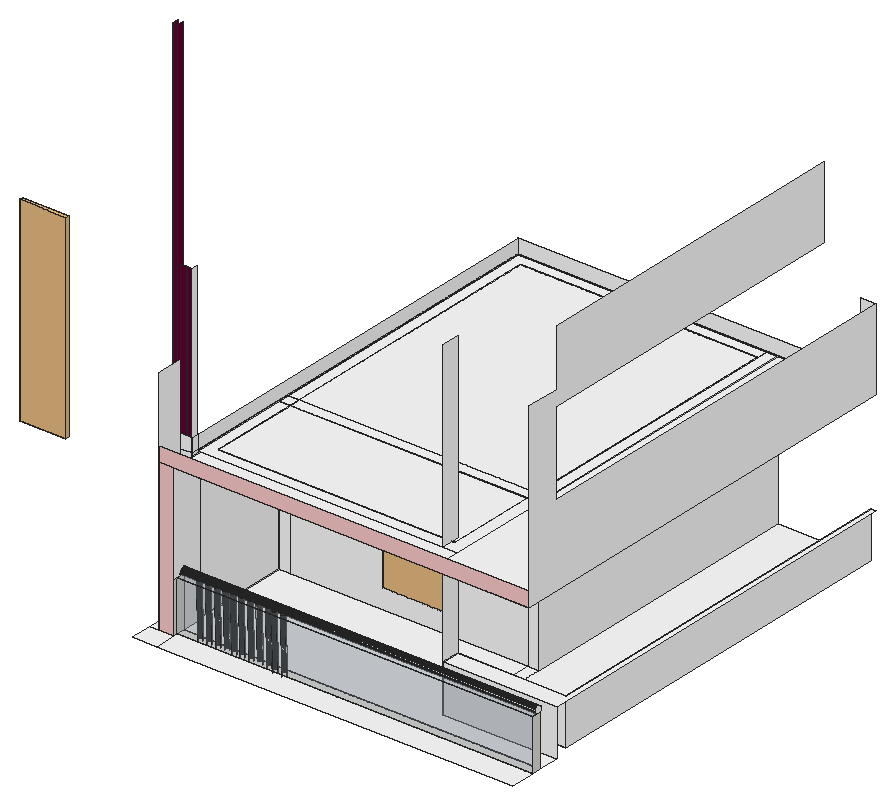
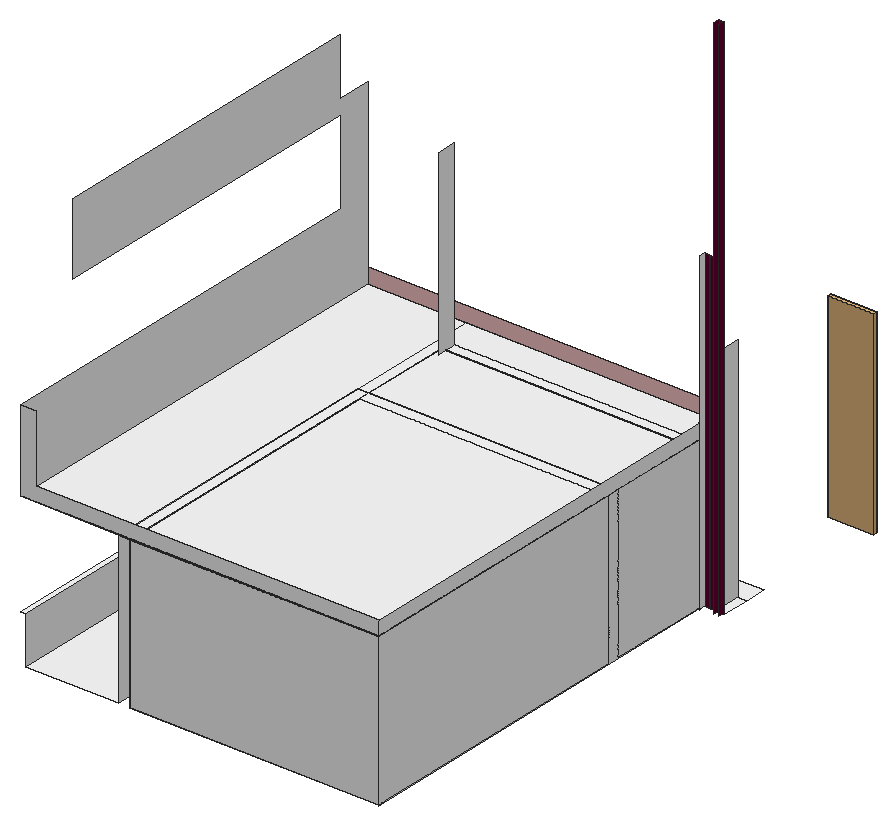
# SketchUp Ruby script. Lengths in inches.
U = 1.inch
M = Sketchup.active_model
def pt(a) = Geom::Point3d.new(a.map { |v| v * U })
def face(e, loops, mat)
  f = e.add_face(loops[0].map { |a| pt(a) })
  loops[1..].each { |l| e.add_face(l.map { |a| pt(a) }).erase! }
  f.material = f.back_material = mat if mat
  f
end
# faces: each face lists its corners as indices into pts; further lists are holes
def faces(e, pts, list, mat = nil) = list.each { |f| face(e, (f[0].is_a?(Array) ? f : [f]).map { |l| l.map { |i| pts[i] } }, mat) }
# xy, xz, yz: faces in a plane at the given z, y or x. An outline is a flat list of corners, or four numbers for a rectangle; further outlines are holes
def ring(l) = l.size == 4 ? [[l[0], l[1]], [l[2], l[1]], [l[2], l[3]], [l[0], l[3]]] : l.each_slice(2).to_a
def flat(e, list, mat, &to3) = list.each { |f| face(e, (f[0].is_a?(Array) ? f : [f]).map { |l| ring(l).map { |u, v| to3.(u, v) } }, mat) }
def xy(e, z, list, mat = nil) = flat(e, list, mat) { |x, y| [x, y, z] }
def xz(e, y, list, mat = nil) = flat(e, list, mat) { |x, z| [x, y, z] }
def yz(e, x, list, mat = nil) = flat(e, list, mat) { |y, z| [x, y, z] }
def lines(e, pts, list) = list.each { |a, b| e.add_line(pt(pts[a]), pt(pts[b])) }
# prism: a flat outline (further loops are holes) pulled along v
def prism(e, loops, v, mat = nil)
  f = face(e, loops, mat); d = Geom::Vector3d.new(v.map { |x| x * U })
  f.pushpull(f.normal.samedirection?(d) ? d.length : -d.length)
end
def box(e, o, s, mat = nil) = prism(e, [[o, [o[0] + s[0], o[1], o[2]], [o[0] + s[0], o[1] + s[1], o[2]], [o[0], o[1] + s[1], o[2]]]], [0, 0, s[2]], mat)
def at(x, y, z, deg = 0) = Geom::Transformation.translation(pt([x, y, z])) * Geom::Transformation.rotation(ORIGIN, Z_AXIS, deg.degrees)
def axes(o, x, y, z) = Geom::Transformation.new([*x, 0, *y, 0, *z, 0, *pt(o).to_a, 1])
def part(name) = M.definitions.add(name)
# library, detail: a bought-in or finely detailed component or shape, given as its bounding box
def library(name, o, s) = part(name).tap { |d| box(d.entities, o, s) }
def detail(e, o, s) = box(e.add_group.entities, o, s)
def put(e, d, t, mat = nil) = e.add_instance(d, t).tap { |i| i.material = mat if mat }
def group(e, t, mat = nil) = e.add_group.tap { |g| g.transformation = t; g.material = mat if mat }.entities
root = M.entities
M.materials.add("A01_Blush_Petal").color = [255, 204, 204]
M.materials.add("Glass_Basic_01").color = [161, 173, 186]
M.materials["Glass_Basic_01"].alpha = 0.25
M.materials.add("L08_Velvet_Rose").color = [102, 0, 51]
M.materials.add("M00_Soft_Cloud").color = [255, 255, 255]
c1 = library("Group\#30",[0,0,0],[77.46,3.16,80.98])
c2 = library("Window 109 023",[-16.24,-1.39,-0.03],[32.48,2.78,89.27])
xy(root,129.83,[[380.49,253.62,393.98,274.78]],"M00_Soft_Cloud")
xy(root,132,[[201,139.66,484.6,146.72]])
xy(root,132,[[182.05,119.76,201,136.44],[201,119.76,484.6,139.66],[182.05,136.44,189,157.97],[189,136.44,189,157.97,199,157.97,199,162.91,201,162.91,201,136.44],[201,146.72,484.6,146.72,484.6,163.42,394.03,163.42,394.03,178.61,396.98,178.61,396.98,244.18,199,244.18,199,162.91,201,162.91],
  [182.05,157.97,183,158.3],[183,157.97,187,158.3],[187,157.97,199,157.97,199,162.91,198,162.91,198,158.3,187,158.3],[396.98,178.61,405.98,244.18],[405.98,178.61,480.39,482.39],
  [199,253.18,208,253.18,208,473.39,396.98,473.39,396.98,482.39,199,482.39],[208,253.18,396.98,473.39]],"M00_Soft_Cloud")
xy(root,169.29,[[394.03,163.42,484.6,163.42,484.6,482.39,480.39,482.39,480.39,178.61,394.03,178.61]],"M00_Soft_Cloud")
xy(root,172.19,[[201,139.66,484.6,146.72]],"Glass_Basic_01")
xy(root,172.25,[[199.77,145.625,484.6,145.65]],"M00_Soft_Cloud")
xy(root,252,[[201,136.44,405.98,162.91],[405.98,136.44,484.6,482.39],[199,162.91,405.98,162.91,405.98,244.18,396.98,244.18,396.98,171.91,208,171.91,208,244.18,199,244.18],[208,171.91,396.98,244.18],[199,244.18,208,253.18],
  [208,244.18,396.98,253.18],[396.98,244.18,405.98,482.39],[199,253.18,208,253.18,208,473.39,396.98,473.39,396.98,482.39,199,482.39],[208,253.18,396.98,473.39]],"M00_Soft_Cloud")
xz(root,136.44,[[189,132,201,252],[189,252,484.6,264]],"A01_Blush_Petal")
xz(root,139.66,[[201,132,484.6,172.19]],"Glass_Basic_01")
xz(root,146.72,[[201,132,484.6,172.19]],"Glass_Basic_01")
xz(root,157.97,[[189,132,199,252.48],[189,252.48,199,263.52]],"M00_Soft_Cloud")
xz(root,158.3,[[183,132,187,554.29],[189,132,193,384],[195,132,198,384]],"L08_Velvet_Rose")
xz(root,162.91,[[198,131.52,199,132],[198,132,199,264.48],[199,132,201,252]],"M00_Soft_Cloud")
xz(root,163.42,[[394.03,132,484.6,169.29]],"M00_Soft_Cloud")
xz(root,178.61,[[394.03,132,480.39,169.29]],"M00_Soft_Cloud")
xz(root,244.18,[[199,132,208,252],[[208,132,396.98,252],[281.67,147.52,339.66,216]],[396.98,132,405.98,252]],"M00_Soft_Cloud")
xz(root,253.18,[[199,132,208,252]],"M00_Soft_Cloud")
xz(root,482.39,[[199,132,396.98,252],[199,252,484.6,252.48],[199,252.48,199,264,472.6,264,472.6,317.36,484.6,317.36,484.6,252.48]],"M00_Soft_Cloud")
yz(root,183,[[158.3,132,162.91,554.29]],"L08_Velvet_Rose")
yz(root,187,[[158.3,132,162.91,554.29]],"L08_Velvet_Rose")
yz(root,189,[[136.44,132,157.97,315.86]],"M00_Soft_Cloud")
yz(root,198,[[158.3,132,162.91,384]],"M00_Soft_Cloud")
yz(root,199,[[162.91,131.52,482.39,131.52,482.39,132,253.18,132,253.18,252,244.18,252,244.18,132,162.91,132],[157.97,132,162.91,252.48],[162.91,132,244.18,252],[253.18,132,482.39,252],[162.91,252,482.39,252.48],
  [157.97,252.48,162.91,263.52],[162.91,252.48,482.39,263.52]],"M00_Soft_Cloud")
yz(root,199.77,[[145.625,172.25,144.9,172.34,144.23,172.62,143.65,173.0625,143.2,173.64,142.93,174.32,142.83,175.04,142.93,175.76,143.2,176.4375,143.65,177.02,144.23,177.46,144.9,177.74,145.625,177.83,146.35,177.74,147.02,177.46,147.6,177.02,148.04,176.4375,148.32,175.76,148.42,175.04,148.32,174.32,148.04,173.64,147.6,173.0625,147.02,172.62,146.35,172.34,145.65,172.25]],"M00_Soft_Cloud")
yz(root,201,[[136.44,132,139.66,172.19],[139.66,132,146.72,172.19]])
yz(root,201,[[146.72,132,162.91,132,162.91,252,136.44,252,136.44,172.19,146.72,172.19]],"M00_Soft_Cloud")
yz(root,394.03,[[163.42,132,178.61,169.29],[163.42,169.29,178.61,396]],"M00_Soft_Cloud")
yz(root,396.98,[[253.18,132,473.39,252],[473.39,132,482.39,252]],"M00_Soft_Cloud")
yz(root,405.98,[[244.18,132,482.39,252]],"M00_Soft_Cloud")
yz(root,480.39,[[178.61,132,482.39,169.29]],"M00_Soft_Cloud")
yz(root,484.6,[[139.66,132,146.72,172.19]])
yz(root,484.6,[[145.625,172.25,145.65,172.25,146.35,172.34,147.02,172.62,147.6,173.0625,148.04,173.64,148.32,174.32,148.42,175.04,148.32,175.76,148.04,176.4375,147.6,177.02,147.02,177.46,146.35,177.74,145.625,177.83,144.9,177.74,144.23,177.46,143.65,177.02,143.2,176.4375,142.93,175.76,142.83,175.04,142.93,174.32,143.2,173.64,143.65,173.0625,144.23,172.62,144.9,172.34],[136.44,252,482.39,252,482.39,317.36,162.91,317.36,162.91,384,429.82,384,429.82,441.51,163.42,441.51,163.42,396,136.44,396]],"M00_Soft_Cloud")
p = [[274.26,142.76,172.56],[274.26,143.97,127.76],[274.64,143.8125,127.76],[274.64,142.61,172.55],[275.06,143.76,127.76],[275.06,142.55,172.55],
  [275.47,143.8125,127.76],[275.47,142.61,172.55],[275.85,143.97,127.76],[275.85,142.76,172.56],[281.27,142.76,172.56],[281.27,143.97,127.76],
  [281.66,143.8125,127.76],[281.66,142.61,172.55],[282.07,143.76,127.76],[282.07,142.55,172.55],[282.48,143.8125,127.76],[282.48,142.61,172.55],
  [282.87,143.97,127.76],[282.87,142.76,172.56],[273.93,143.02,172.5625],[273.93,144.23,127.76],[276.1875,144.23,127.76],[276.1875,143.02,172.5625],
  [280.94,143.02,172.5625],[280.94,144.23,127.76],[283.2,144.23,127.76],[283.2,143.02,172.5625],[273.67,143.35,172.57],[273.67,144.56,127.76],
  [276.4375,144.56,127.76],[276.4375,143.35,172.57],[280.6875,143.35,172.57],[280.6875,144.56,127.76],[283.45,144.56,127.76],[283.45,143.35,172.57],
  [273.51,143.73,172.58],[273.51,144.94,127.76],[276.6,144.94,127.76],[276.6,143.73,172.58],[280.53,143.73,172.58],[280.53,144.94,127.76],
  [283.61,144.94,127.76],[283.61,143.73,172.58],[273.46,144.15,172.59],[273.46,145.36,127.76],[276.65,145.36,127.76],[276.65,144.15,172.59],
  [280.47,144.15,172.59],[280.47,145.36,127.76],[283.67,145.36,127.76],[283.67,144.15,172.59],[273.51,145.77,127.77],[273.51,144.5625,172.6],
  [276.6,145.77,127.77],[276.6,144.5625,172.6],[280.53,145.77,127.77],[280.53,144.5625,172.6],[283.61,145.77,127.77],[283.61,144.5625,172.6],
  [273.67,146.16,127.78],[273.67,144.95,172.62],[276.4375,146.16,127.78],[276.4375,144.95,172.62],[280.6875,146.16,127.78],[280.6875,144.95,172.62],
  [283.45,146.16,127.78],[283.45,144.95,172.62],[273.93,146.49,127.79],[273.93,145.28,172.625],[276.1875,146.49,127.79],[276.1875,145.28,172.625],
  [280.94,146.49,127.79],[280.94,145.28,172.625],[283.2,146.49,127.79],[283.2,145.28,172.625],[274.26,146.74,127.8],[274.26,145.53,172.63],
  [275.85,146.74,127.8],[275.85,145.53,172.63],[281.27,146.74,127.8],[281.27,145.53,172.63],[282.87,146.74,127.8],[282.87,145.53,172.63],
  [274.64,146.9,127.8],[274.64,145.69,172.64],[275.47,146.9,127.8],[275.47,145.69,172.64],[281.66,146.9,127.8],[281.66,145.69,172.64],
  [282.48,146.9,127.8],[282.48,145.69,172.64],[275.06,146.95,127.8],[275.06,145.74,172.64],[282.07,146.95,127.8],[282.07,145.74,172.64],
  [213.7,144.08,173.3],[213.7,145.29,128.5],[214.11,145.24,128.5],[214.11,144.03,173.29],[214.52,145.29,128.5],[214.52,144.08,173.3],
  [220.82,144.08,173.3],[220.82,145.29,128.5],[221.23,145.24,128.5],[221.23,144.03,173.29],[221.65,145.29,128.5],[221.65,144.08,173.3],
  [228.125,144.08,173.3],[228.125,145.29,128.5],[228.54,145.24,128.5],[228.54,144.03,173.29],[228.95,145.29,128.5],[228.95,144.08,173.3],
  [234.86,144.08,173.3],[234.86,145.29,128.5],[235.28,145.24,128.5],[235.28,144.03,173.29],[235.69,145.29,128.5],[235.69,144.08,173.3],
  [240.71,144.08,173.3],[240.71,145.29,128.5],[241.125,145.24,128.5],[241.125,144.03,173.29],[241.54,145.29,128.5],[241.54,144.08,173.3],
  [247.37,144.08,173.3],[247.37,145.29,128.5],[247.78,145.24,128.5],[247.78,144.03,173.29],[248.19,145.29,128.5],[248.19,144.08,173.3],
  [254.26,144.08,173.3],[254.26,145.29,128.5],[254.68,145.24,128.5],[254.68,144.03,173.29],[255.09,145.29,128.5],[255.09,144.08,173.3],
  [261.2,144.08,173.3],[261.2,145.29,128.5],[261.61,145.24,128.5],[261.61,144.03,173.29],[262.03,145.29,128.5],[262.03,144.08,173.3],
  [268.52,144.08,173.3],[268.52,145.29,128.5],[268.93,145.24,128.5],[268.93,144.03,173.29],[269.35,145.29,128.5],[269.35,144.08,173.3],
  [213.3125,144.24,173.3],[213.3125,145.45,128.5],[214.91,145.45,128.5],[214.91,144.24,173.3],[220.43,144.24,173.3],[220.43,145.45,128.5],
  [222.03,145.45,128.5],[222.03,144.24,173.3],[227.74,144.24,173.3],[227.74,145.45,128.5],[229.34,145.45,128.5],[229.34,144.24,173.3],
  [234.48,144.24,173.3],[234.48,145.45,128.5],[236.08,145.45,128.5],[236.08,144.24,173.3],[240.33,144.24,173.3],[240.33,145.45,128.5],
  [241.93,145.45,128.5],[241.93,144.24,173.3],[246.98,144.24,173.3],[246.98,145.45,128.5],[248.58,145.45,128.5],[248.58,144.24,173.3],
  [253.88,144.24,173.3],[253.88,145.45,128.5],[255.48,145.45,128.5],[255.48,144.24,173.3],[260.82,144.24,173.3],[260.82,145.45,128.5],
  [262.41,145.45,128.5],[262.41,144.24,173.3],[268.14,144.24,173.3],[268.14,145.45,128.5],[269.73,145.45,128.5],[269.73,144.24,173.3],
  [212.98,144.49,173.31],[212.98,145.7,128.5],[215.24,145.7,128.5],[215.24,144.49,173.31],[220.1,144.49,173.31],[220.1,145.7,128.5],
  [222.36,145.7,128.5],[222.36,144.49,173.31],[227.41,144.49,173.31],[227.41,145.7,128.5],[229.67,145.7,128.5],[229.67,144.49,173.31],
  [234.15,144.49,173.31],[234.15,145.7,128.5],[236.41,145.7,128.5],[236.41,144.49,173.31],[240,144.49,173.31],[240,145.7,128.5],
  [242.26,145.7,128.5],[242.26,144.49,173.31],[246.65,144.49,173.31],[246.65,145.7,128.5],[248.91,145.7,128.5],[248.91,144.49,173.31],
  [253.55,144.49,173.31],[253.55,145.7,128.5],[255.81,145.7,128.5],[255.81,144.49,173.31],[260.48,144.49,173.31],[260.48,145.7,128.5],
  [262.74,145.7,128.5],[262.74,144.49,173.31],[267.8,144.49,173.31],[267.8,145.7,128.5],[270.0625,145.7,128.5],[270.0625,144.49,173.31],
  [212.73,144.83,173.32],[212.73,146.03,128.5],[215.49,146.03,128.5],[215.49,144.83,173.32],[219.85,144.83,173.32],[219.85,146.03,128.5],
  [222.62,146.03,128.5],[222.62,144.83,173.32],[227.15,144.83,173.32],[227.15,146.03,128.5],[229.92,146.03,128.5],[229.92,144.83,173.32],
  [233.89,144.83,173.32],[233.89,146.03,128.5],[236.66,146.03,128.5],[236.66,144.83,173.32],[239.74,144.83,173.32],[239.74,146.03,128.5],
  [242.51,146.03,128.5],[242.51,144.83,173.32],[246.4,144.83,173.32],[246.4,146.03,128.5],[249.16,146.03,128.5],[249.16,144.83,173.32],
  [253.29,144.83,173.32],[253.29,146.03,128.5],[256.06,146.03,128.5],[256.06,144.83,173.32],[260.23,144.83,173.32],[260.23,146.03,128.5],
  [263,146.03,128.5],[263,144.83,173.32],[267.55,144.83,173.32],[267.55,146.03,128.5],[270.32,146.03,128.5],[270.32,144.83,173.32],
  [212.57,145.21,173.33],[212.57,146.42,128.5],[215.65,146.42,128.5],[215.65,145.21,173.33],[219.69,145.21,173.33],[219.69,146.42,128.5],
  [222.78,146.42,128.5],[222.78,145.21,173.33],[227,145.21,173.33],[227,146.42,128.5],[230.08,146.42,128.5],[230.08,145.21,173.33],
  [233.73,145.21,173.33],[233.73,146.42,128.5],[236.82,146.42,128.5],[236.82,145.21,173.33],[239.58,145.21,173.33],[239.58,146.42,128.5],
  [242.67,146.42,128.5],[242.67,145.21,173.33],[246.24,145.21,173.33],[246.24,146.42,128.5],[249.32,146.42,128.5],[249.32,145.21,173.33],
  [253.13,145.21,173.33],[253.13,146.42,128.5],[256.22,146.42,128.5],[256.22,145.21,173.33],[260.07,145.21,173.33],[260.07,146.42,128.5],
  [263.16,146.42,128.5],[263.16,145.21,173.33],[267.39,145.21,173.33],[267.39,146.42,128.5],[270.48,146.42,128.5],[270.48,145.21,173.33],
  [212.51,145.65,172.25],[212.51,146.83,128.5],[212.51,145.625,173.34],[215.71,146.83,128.5],[215.71,145.65,172.25],[215.71,145.625,173.34],
  [219.64,145.65,172.25],[219.64,146.83,128.5],[219.64,145.625,173.34],[222.83,146.83,128.5],[222.83,145.65,172.25],[222.83,145.625,173.34],
  [226.94,145.65,172.25],[226.94,146.83,128.5],[226.94,145.625,173.34],[230.14,146.83,128.5],[230.14,145.65,172.25],[230.14,145.625,173.34],
  [233.68,145.65,172.25],[233.68,146.83,128.5],[233.68,145.625,173.34],[236.875,146.83,128.5],[236.875,145.65,172.25],[236.875,145.625,173.34],
  [239.53,145.65,172.25],[239.53,146.83,128.5],[239.53,145.625,173.34],[242.72,146.83,128.5],[242.72,145.65,172.25],[242.72,145.625,173.34],
  [246.18,145.65,172.25],[246.18,146.83,128.5],[246.18,145.625,173.34],[249.38,146.83,128.5],[249.38,145.65,172.25],[249.38,145.625,173.34],
  [253.08,145.65,172.25],[253.08,146.83,128.5],[253.08,145.625,173.34],[256.27,146.83,128.5],[256.27,145.65,172.25],[256.27,145.625,173.34],
  [260.02,145.65,172.25],[260.02,146.83,128.5],[260.02,145.625,173.34],[263.21,146.83,128.5],[263.21,145.65,172.25],[263.21,145.625,173.34],
  [267.34,145.65,172.25],[267.34,146.83,128.5],[267.34,145.625,173.34],[270.53,146.83,128.5],[270.53,145.65,172.25],[270.53,145.625,173.34],
  [212.57,147.25,128.52],[212.57,146.04,173.35],[215.65,147.25,128.52],[215.65,146.04,173.35],[219.69,147.25,128.52],[219.69,146.04,173.35],
  [222.78,147.25,128.52],[222.78,146.04,173.35],[227,147.25,128.52],[227,146.04,173.35],[230.08,147.25,128.52],[230.08,146.04,173.35],
  [233.73,147.25,128.52],[233.73,146.04,173.35],[236.82,147.25,128.52],[236.82,146.04,173.35],[239.58,147.25,128.52],[239.58,146.04,173.35],
  [242.67,147.25,128.52],[242.67,146.04,173.35],[246.24,147.25,128.52],[246.24,146.04,173.35],[249.32,147.25,128.52],[249.32,146.04,173.35],
  [253.13,147.25,128.52],[253.13,146.04,173.35],[256.22,147.25,128.52],[256.22,146.04,173.35],[260.07,147.25,128.52],[260.07,146.04,173.35],
  [263.16,147.25,128.52],[263.16,146.04,173.35],[267.39,147.25,128.52],[267.39,146.04,173.35],[270.48,147.25,128.52],[270.48,146.04,173.35],
  [212.73,147.63,128.53],[212.73,146.42,173.36],[215.49,147.63,128.53],[215.49,146.42,173.36],[219.85,147.63,128.53],[219.85,146.42,173.36],
  [222.62,147.63,128.53],[222.62,146.42,173.36],[227.15,147.63,128.53],[227.15,146.42,173.36],[229.92,147.63,128.53],[229.92,146.42,173.36],
  [233.89,147.63,128.53],[233.89,146.42,173.36],[236.66,147.63,128.53],[236.66,146.42,173.36],[239.74,147.63,128.53],[239.74,146.42,173.36],
  [242.51,147.63,128.53],[242.51,146.42,173.36],[246.4,147.63,128.53],[246.4,146.42,173.36],[249.16,147.63,128.53],[249.16,146.42,173.36],
  [253.29,147.63,128.53],[253.29,146.42,173.36],[256.06,147.63,128.53],[256.06,146.42,173.36],[260.23,147.63,128.53],[260.23,146.42,173.36],
  [263,147.63,128.53],[263,146.42,173.36],[267.55,147.63,128.53],[267.55,146.42,173.36],[270.32,147.63,128.53],[270.32,146.42,173.36],
  [212.98,147.96,128.54],[212.98,146.75,173.37],[215.24,147.96,128.54],[215.24,146.75,173.37],[220.1,147.96,128.54],[220.1,146.75,173.37],
  [222.36,147.96,128.54],[222.36,146.75,173.37],[227.41,147.96,128.54],[227.41,146.75,173.37],[229.67,147.96,128.54],[229.67,146.75,173.37],
  [234.15,147.96,128.54],[234.15,146.75,173.37],[236.41,147.96,128.54],[236.41,146.75,173.37],[240,147.96,128.54],[240,146.75,173.37],
  [242.26,147.96,128.54],[242.26,146.75,173.37],[246.65,147.96,128.54],[246.65,146.75,173.37],[248.91,147.96,128.54],[248.91,146.75,173.37],
  [253.55,147.96,128.54],[253.55,146.75,173.37],[255.81,147.96,128.54],[255.81,146.75,173.37],[260.48,147.96,128.54],[260.48,146.75,173.37],
  [262.74,147.96,128.54],[262.74,146.75,173.37],[267.8,147.96,128.54],[267.8,146.75,173.37],[270.0625,147.96,128.54],[270.0625,146.75,173.37],
  [213.3125,148.22,128.54],[213.3125,147.01,173.375],[214.91,148.22,128.54],[214.91,147.01,173.375],[220.43,148.22,128.54],[220.43,147.01,173.375],
  [222.03,148.22,128.54],[222.03,147.01,173.375],[227.74,148.22,128.54],[227.74,147.01,173.375],[229.34,148.22,128.54],[229.34,147.01,173.375],
  [234.48,148.22,128.54],[234.48,147.01,173.375],[236.08,148.22,128.54],[236.08,147.01,173.375],[240.33,148.22,128.54],[240.33,147.01,173.375],
  [241.93,148.22,128.54],[241.93,147.01,173.375],[246.98,148.22,128.54],[246.98,147.01,173.375],[248.58,148.22,128.54],[248.58,147.01,173.375],
  [253.88,148.22,128.54],[253.88,147.01,173.375],[255.48,148.22,128.54],[255.48,147.01,173.375],[260.82,148.22,128.54],[260.82,147.01,173.375],
  [262.41,148.22,128.54],[262.41,147.01,173.375],[268.14,148.22,128.54],[268.14,147.01,173.375],[269.73,148.22,128.54],[269.73,147.01,173.375],
  [213.7,148.375,128.55],[213.7,147.17,173.38],[214.52,148.375,128.55],[214.52,147.17,173.38],[220.82,148.375,128.55],[220.82,147.17,173.38],
  [221.65,148.375,128.55],[221.65,147.17,173.38],[228.125,148.375,128.55],[228.125,147.17,173.38],[228.95,148.375,128.55],[228.95,147.17,173.38],
  [234.86,148.375,128.55],[234.86,147.17,173.38],[235.69,148.375,128.55],[235.69,147.17,173.38],[240.71,148.375,128.55],[240.71,147.17,173.38],
  [241.54,148.375,128.55],[241.54,147.17,173.38],[247.37,148.375,128.55],[247.37,147.17,173.38],[248.19,148.375,128.55],[248.19,147.17,173.38],
  [254.26,148.375,128.55],[254.26,147.17,173.38],[255.09,148.375,128.55],[255.09,147.17,173.38],[261.2,148.375,128.55],[261.2,147.17,173.38],
  [262.03,148.375,128.55],[262.03,147.17,173.38],[268.52,148.375,128.55],[268.52,147.17,173.38],[269.35,148.375,128.55],[269.35,147.17,173.38],
  [214.11,148.43,128.55],[214.11,147.22,173.38],[221.23,148.43,128.55],[221.23,147.22,173.38],[228.54,148.43,128.55],[228.54,147.22,173.38],
  [235.28,148.43,128.55],[235.28,147.22,173.38],[241.125,148.43,128.55],[241.125,147.22,173.38],[247.78,148.43,128.55],[247.78,147.22,173.38],
  [254.68,148.43,128.55],[254.68,147.22,173.38],[261.61,148.43,128.55],[261.61,147.22,173.38],[268.93,148.43,128.55],[268.93,147.22,173.38],
  [484.6,144.9,172.34],[199.77,144.9,172.34],[199.77,145.625,172.25],[484.6,145.625,172.25],[484.6,144.23,172.62],[199.77,144.23,172.62],
  [199.77,145.65,172.25],[199.77,146.35,172.34],[484.6,146.35,172.34],[484.6,145.65,172.25],[199.77,147.02,172.62],[484.6,147.02,172.62],
  [484.6,143.65,173.0625],[199.77,143.65,173.0625],[199.77,147.6,173.0625],[484.6,147.6,173.0625],[484.6,143.2,173.64],[199.77,143.2,173.64],
  [199.77,148.04,173.64],[484.6,148.04,173.64],[484.6,142.93,174.32],[199.77,142.93,174.32],[199.77,148.32,174.32],[484.6,148.32,174.32],
  [484.6,142.83,175.04],[199.77,142.83,175.04],[199.77,148.42,175.04],[484.6,148.42,175.04],[484.6,142.93,175.76],[199.77,142.93,175.76],
  [199.77,148.32,175.76],[484.6,148.32,175.76],[484.6,143.2,176.4375],[199.77,143.2,176.4375],[199.77,148.04,176.4375],[484.6,148.04,176.4375],
  [484.6,143.65,177.02],[199.77,143.65,177.02],[199.77,147.6,177.02],[484.6,147.6,177.02],[484.6,144.23,177.46],[199.77,144.23,177.46],
  [199.77,147.02,177.46],[484.6,147.02,177.46],[484.6,144.9,177.74],[199.77,144.9,177.74],[199.77,146.35,177.74],[484.6,146.35,177.74],
  [484.6,145.625,177.83],[199.77,145.625,177.83],[208,473.39,252.48],[208,171.91,252.48],[396.98,171.91,252.48],[396.98,473.39,252.48],
  [396.98,171.91,132],[396.98,171.91,132.48],[396.98,178.61,132],[463.64,144.39,174.27],[463.64,144.33,174.68],[463.64,144.55,173.88],
  [463.64,144.39,175.09],[463.64,144.55,175.48],[463.64,144.8,175.8125],[463.64,145.13,176.06],[463.64,146.73,173.3],[463.64,146.34,173.14],
  [463.64,145.93,173.08],[463.64,147.47,174.27],[463.64,147.3125,173.88],[463.64,145.13,173.3],[463.64,144.8,173.55],[463.64,147.53,174.68],
  [463.64,147.06,173.55],[463.64,145.52,173.14],[199.04,144.55,175.48],[199.04,144.39,175.09],[199.04,144.33,174.68],[199.04,144.39,174.27],
  [199.04,145.93,173.08],[199.04,146.34,173.14],[199.04,146.73,173.3],[199.04,147.06,173.55],[199.04,147.3125,173.88],[199.04,147.47,174.27],
  [199.04,147.53,174.68],[199.04,145.52,173.14],[199.04,147.47,175.09],[199.04,144.8,175.8125],[199.04,145.13,176.06],[199.04,145.13,173.3],
  [199.04,144.55,173.88],[199.04,144.8,173.55],[199.04,145.52,176.22],[463.64,147.06,175.8125],[463.64,147.3125,175.48],[199.04,147.3125,175.48],
  [199.04,147.06,175.8125],[199.04,145.93,176.28],[463.64,145.52,176.22],[463.64,147.47,175.09],[463.64,146.34,176.22],[463.64,146.73,176.06],
  [199.04,146.34,176.22],[463.64,145.93,176.28],[199.04,146.73,176.06],[405.98,162.91,132],[405.98,162.91,132.37],[405.98,162.91,132.48]]
faces(root,p,[[0,1,2,3],[3,2,4,5],[5,4,6,7],[7,6,8,9],[10,11,12,13],[13,12,14,15],[15,14,16,17],[17,16,18,19],
  [20,21,1,0],[9,8,22,23],[24,25,11,10],[19,18,26,27],[28,29,21,20],[23,22,30,31],[32,33,25,24],[27,26,34,35],
  [36,37,29,28],[31,30,38,39],[40,41,33,32],[35,34,42,43],[44,45,37,36],[39,38,46,47],[48,49,41,40],[43,42,50,51],
  [52,45,44,53],[46,54,55,47],[56,49,48,57],[50,58,59,51],[60,52,53,61],[54,62,63,55],[64,56,57,65],[58,66,67,59],
  [68,60,61,69],[62,70,71,63],[72,64,65,73],[66,74,75,67],[76,68,69,77],[70,78,79,71],[80,72,73,81],[74,82,83,75],
  [84,76,77,85],[78,86,87,79],[88,80,81,89],[82,90,91,83],[92,84,85,93],[86,92,93,87],[94,88,89,95],[90,94,95,91],
  [96,97,98,99],[99,98,100,101],[102,103,104,105],[105,104,106,107],[108,109,110,111],[111,110,112,113],[114,115,116,117],[117,116,118,119],
  [120,121,122,123],[123,122,124,125],[126,127,128,129],[129,128,130,131],[132,133,134,135],[135,134,136,137],[138,139,140,141],[141,140,142,143],
  [144,145,146,147],[147,146,148,149],[150,151,97,96],[101,100,152,153],[154,155,103,102],[107,106,156,157],[158,159,109,108],[113,112,160,161],
  [162,163,115,114],[119,118,164,165],[166,167,121,120],[125,124,168,169],[170,171,127,126],[131,130,172,173],[174,175,133,132],[137,136,176,177],
  [178,179,139,138],[143,142,180,181],[182,183,145,144],[149,148,184,185],[186,187,151,150],[153,152,188,189],[190,191,155,154],[157,156,192,193],
  [194,195,159,158],[161,160,196,197],[198,199,163,162],[165,164,200,201],[202,203,167,166],[169,168,204,205],[206,207,171,170],[173,172,208,209],
  [210,211,175,174],[177,176,212,213],[214,215,179,178],[181,180,216,217],[218,219,183,182],[185,184,220,221],[222,223,187,186],[189,188,224,225],
  [226,227,191,190],[193,192,228,229],[230,231,195,194],[197,196,232,233],[234,235,199,198],[201,200,236,237],[238,239,203,202],[205,204,240,241],
  [242,243,207,206],[209,208,244,245],[246,247,211,210],[213,212,248,249],[250,251,215,214],[217,216,252,253],[254,255,219,218],[221,220,256,257],
  [258,259,223,222],[225,224,260,261],[262,263,227,226],[229,228,264,265],[266,267,231,230],[233,232,268,269],[270,271,235,234],[237,236,272,273],
  [274,275,239,238],[241,240,276,277],[278,279,243,242],[245,244,280,281],[282,283,247,246],[249,248,284,285],[286,287,251,250],[253,252,288,289],
  [290,291,255,254],[257,256,292,293],[294,295,259,258,296],[261,260,297,298,299],[300,301,263,262,302],[265,264,303,304,305],[306,307,267,266,308],[269,268,309,310,311],
  [312,313,271,270,314],[273,272,315,316,317],[318,319,275,274,320],[277,276,321,322,323],[324,325,279,278,326],[281,280,327,328,329],[330,331,283,282,332],[285,284,333,334,335],
  [336,337,287,286,338],[289,288,339,340,341],[342,343,291,290,344],[293,292,345,346,347],[348,295,294,296,349],[297,350,351,299,298],[352,301,300,302,353],[303,354,355,305,304],
  [356,307,306,308,357],[309,358,359,311,310],[360,313,312,314,361],[315,362,363,317,316],[364,319,318,320,365],[321,366,367,323,322],[368,325,324,326,369],[327,370,371,329,328],
  [372,331,330,332,373],[333,374,375,335,334],[376,337,336,338,377],[339,378,379,341,340],[380,343,342,344,381],[345,382,383,347,346],[384,348,349,385],[350,386,387,351],
  [388,352,353,389],[354,390,391,355],[392,356,357,393],[358,394,395,359],[396,360,361,397],[362,398,399,363],[400,364,365,401],[366,402,403,367],
  [404,368,369,405],[370,406,407,371],[408,372,373,409],[374,410,411,375],[412,376,377,413],[378,414,415,379],[416,380,381,417],[382,418,419,383],
  [420,384,385,421],[386,422,423,387],[424,388,389,425],[390,426,427,391],[428,392,393,429],[394,430,431,395],[432,396,397,433],[398,434,435,399],
  [436,400,401,437],[402,438,439,403],[440,404,405,441],[406,442,443,407],[444,408,409,445],[410,446,447,411],[448,412,413,449],[414,450,451,415],
  [452,416,417,453],[418,454,455,419],[456,420,421,457],[422,458,459,423],[460,424,425,461],[426,462,463,427],[464,428,429,465],[430,466,467,431],
  [468,432,433,469],[434,470,471,435],[472,436,437,473],[438,474,475,439],[476,440,441,477],[442,478,479,443],[480,444,445,481],[446,482,483,447],
  [484,448,449,485],[450,486,487,451],[488,452,453,489],[454,490,491,455],[492,456,457,493],[458,494,495,459],[496,460,461,497],[462,498,499,463],
  [500,464,465,501],[466,502,503,467],[504,468,469,505],[470,506,507,471],[508,472,473,509],[474,510,511,475],[512,476,477,513],[478,514,515,479],
  [516,480,481,517],[482,518,519,483],[520,484,485,521],[486,522,523,487],[524,488,489,525],[490,526,527,491],[528,492,493,529],[494,528,529,495],
  [530,496,497,531],[498,530,531,499],[532,500,501,533],[502,532,533,503],[534,504,505,535],[506,534,535,507],[536,508,509,537],[510,536,537,511],
  [538,512,513,539],[514,538,539,515],[540,516,517,541],[518,540,541,519],[542,520,521,543],[522,542,543,523],[544,524,525,545],[526,544,545,527],
  [546,547,548,549],[550,551,547,546],[298,294,552,553,554,555,346,342,340,336,334,330,328,324,322,318,316,312,310,306,304,300],[554,553,556,557],[558,559,551,550],[557,556,560,561],[562,563,559,558],[561,560,564,565],
  [566,567,563,562],[565,564,568,569],[570,571,567,566],[569,568,572,573],[574,575,571,570],[573,572,576,577],[578,579,575,574],[577,576,580,581],
  [582,583,579,578],[581,580,584,585],[586,587,583,582],[585,584,588,589],[590,591,587,586],[589,588,592,593],[594,595,591,590],[593,592,595,594]],"M00_Soft_Cloud")
lines(root,p,[[596,597],[597,598],[598,599],[599,596],[600,601],[600,602],[603,604],[605,603],[606,607],[607,608],[608,609],[604,606],
  [610,611],[611,612],[613,614],[615,616],[616,605],[617,613],[614,618],[618,610],[612,619],[619,615],[620,621],[622,623],
  [624,625],[626,627],[627,628],[629,630],[631,624],[630,632],[625,626],[633,620],[621,622],[634,633],[635,631],[623,636],
  [628,629],[637,635],[636,637],[638,634],[639,640],[632,641],[641,642],[643,638],[609,644],[640,645],[646,647],[648,643],
  [649,646],[650,648],[645,617],[642,650],[644,649],[647,639],[651,652],[652,653]])
put(root,c1,axes([281.67,244.18,147.52],[0.7487,0,0],[0,1,0],[0,0,0.84674]))
put(root,c2,axes([82.29,156.3,229.8125],[1.12885,0,0],[0,1.00646,0],[0,0,1.77049]))
